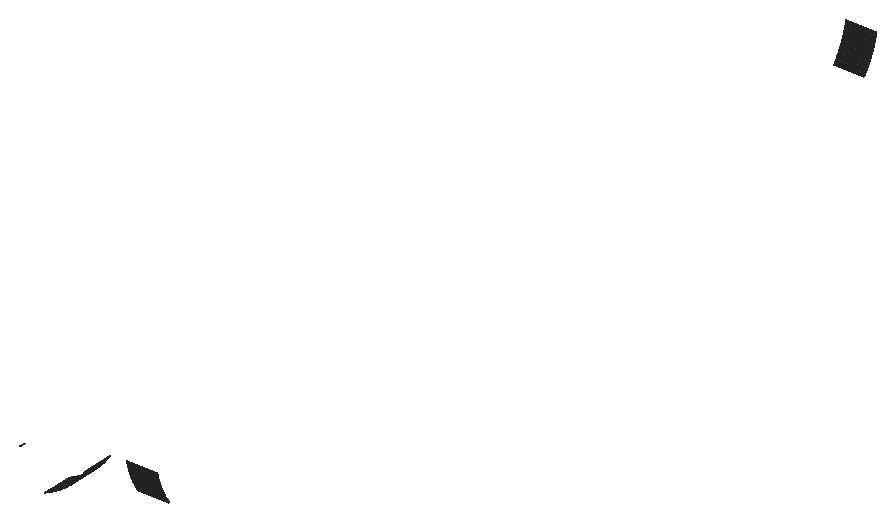
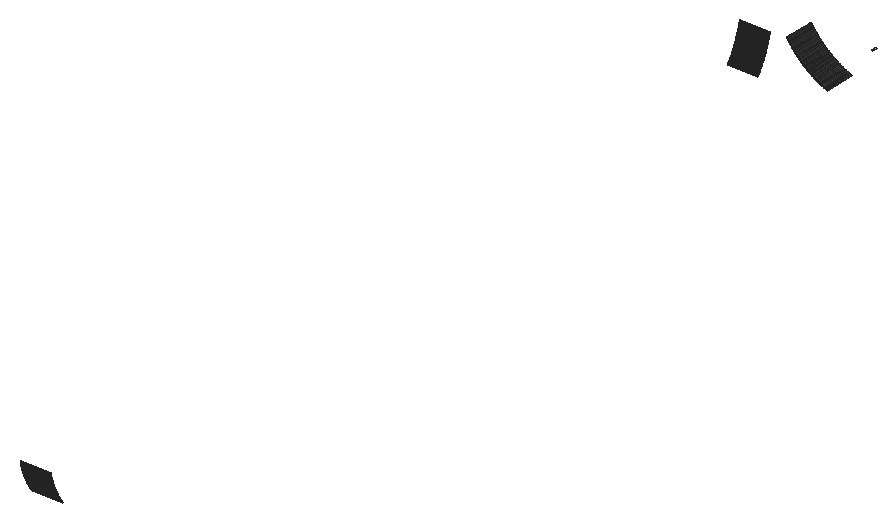
# SketchUp Ruby script. Lengths in inches.
U = 1.inch
M = Sketchup.active_model
def pt(a) = Geom::Point3d.new(a.map { |v| v * U })
def face(e, loops, mat)
  f = e.add_face(loops[0].map { |a| pt(a) })
  loops[1..].each { |l| e.add_face(l.map { |a| pt(a) }).erase! }
  f.material = f.back_material = mat if mat
  f
end
# faces: each face lists its corners as indices into pts; further lists are holes
def faces(e, pts, list, mat = nil) = list.each { |f| face(e, (f[0].is_a?(Array) ? f : [f]).map { |l| l.map { |i| pts[i] } }, mat) }
# xy, xz, yz: faces in a plane at the given z, y or x. An outline is a flat list of corners, or four numbers for a rectangle; further outlines are holes
def ring(l) = l.size == 4 ? [[l[0], l[1]], [l[2], l[1]], [l[2], l[3]], [l[0], l[3]]] : l.each_slice(2).to_a
def flat(e, list, mat, &to3) = list.each { |f| face(e, (f[0].is_a?(Array) ? f : [f]).map { |l| ring(l).map { |u, v| to3.(u, v) } }, mat) }
def xy(e, z, list, mat = nil) = flat(e, list, mat) { |x, y| [x, y, z] }
def xz(e, y, list, mat = nil) = flat(e, list, mat) { |x, z| [x, y, z] }
def yz(e, x, list, mat = nil) = flat(e, list, mat) { |y, z| [x, y, z] }
def lines(e, pts, list) = list.each { |a, b| e.add_line(pt(pts[a]), pt(pts[b])) }
# prism: a flat outline (further loops are holes) pulled along v
def prism(e, loops, v, mat = nil)
  f = face(e, loops, mat); d = Geom::Vector3d.new(v.map { |x| x * U })
  f.pushpull(f.normal.samedirection?(d) ? d.length : -d.length)
end
def box(e, o, s, mat = nil) = prism(e, [[o, [o[0] + s[0], o[1], o[2]], [o[0] + s[0], o[1] + s[1], o[2]], [o[0], o[1] + s[1], o[2]]]], [0, 0, s[2]], mat)
def at(x, y, z, deg = 0) = Geom::Transformation.translation(pt([x, y, z])) * Geom::Transformation.rotation(ORIGIN, Z_AXIS, deg.degrees)
def axes(o, x, y, z) = Geom::Transformation.new([*x, 0, *y, 0, *z, 0, *pt(o).to_a, 1])
def part(name) = M.definitions.add(name)
# library, detail: a bought-in or finely detailed component or shape, given as its bounding box
def library(name, o, s) = part(name).tap { |d| box(d.entities, o, s) }
def detail(e, o, s) = box(e.add_group.entities, o, s)
def put(e, d, t, mat = nil) = e.add_instance(d, t).tap { |i| i.material = mat if mat }
def group(e, t, mat = nil) = e.add_group.tap { |g| g.transformation = t; g.material = mat if mat }.entities
root = M.entities
M.materials.add("1432 AP 8245 TAR ROAD").color = [71, 72, 75]
M.materials.add("Outer Light").color = [251, 217, 152]
p = [[550.51,107.37,158.43],[550.78,107.37,158.53],[550.78,95.37,158.53],[550.51,95.37,158.43],[551.04,107.37,158.64],[551.04,95.37,158.64],
  [551.3,107.37,158.75],[551.3,95.37,158.75],[573,114.08,158.86],[573,114.25,158.63],[585,114.25,158.63],[585,114.08,158.86],
  [573,460.49,158.63],[573,460.66,158.86],[585,460.66,158.86],[585,460.49,158.63],[551.56,107.37,158.87],[551.56,95.37,158.87],
  [551.81,107.37,158.98],[551.81,95.37,158.98],[573,113.92,159.09],[585,113.92,159.09],[573,460.82,159.09],[585,460.82,159.09],
  [552.07,107.37,159.1],[552.07,95.37,159.1],[552.33,107.37,159.22],[552.33,95.37,159.22],[573,113.75,159.32],[585,113.75,159.32],
  [573,460.98,159.32],[585,460.98,159.32],[552.58,107.37,159.34],[552.58,95.37,159.34],[552.84,107.37,159.46],[552.84,95.37,159.46],
  [573,113.6,159.56],[585,113.6,159.56],[573,461.14,159.56],[585,461.14,159.56],[553.09,107.37,159.59],[553.09,95.37,159.59],
  [553.34,107.37,159.72],[553.34,95.37,159.72],[573,113.4375,159.79],[585,113.4375,159.79],[573,461.3,159.79],[585,461.3,159.79],
  [553.6,107.37,159.85],[553.6,95.37,159.85],[553.85,107.37,159.98],[553.85,95.37,159.98],[573,113.28,160.03],[585,113.28,160.03],
  [573,461.46,160.03],[585,461.46,160.03],[554.09,107.37,160.11],[554.09,95.37,160.11],[573,113.125,160.26],[585,113.125,160.26],
  [573,461.61,160.26],[585,461.61,160.26],[554.34,107.37,160.25],[554.34,95.37,160.25],[554.59,107.37,160.38],[554.59,95.37,160.38],
  [573,112.97,160.5],[585,112.97,160.5],[573,461.77,160.5],[585,461.77,160.5],[554.84,107.37,160.52],[554.84,95.37,160.52],
  [555.08,107.37,160.66],[555.08,95.37,160.66],[573,112.82,160.74],[585,112.82,160.74],[573,461.92,160.74],[585,461.92,160.74],
  [555.33,107.37,160.81],[555.33,95.37,160.81],[573,112.67,160.98],[585,112.67,160.98],[573,462.06,160.98],[585,462.06,160.98],
  [555.57,107.37,160.95],[555.57,95.37,160.95],[555.81,107.37,161.1],[555.81,95.37,161.1],[573,112.53,161.22],[585,112.53,161.22],
  [573,462.21,161.22],[585,462.21,161.22],[556.05,107.37,161.25],[556.05,95.37,161.25],[556.29,107.37,161.4],[556.29,95.37,161.4],
  [573,112.38,161.47],[585,112.38,161.47],[573,462.36,161.47],[585,462.36,161.47],[556.53,107.37,161.55],[556.53,95.37,161.55],
  [556.76,107.37,161.7],[556.76,95.37,161.7],[573,112.24,161.71],[585,112.24,161.71],[573,462.5,161.71],[585,462.5,161.71],
  [557,107.37,161.86],[557,95.37,161.86],[573,112.1,161.96],[585,112.1,161.96],[573,462.64,161.96],[585,462.64,161.96],
  [557.24,107.37,162.02],[557.24,95.37,162.02],[557.47,107.37,162.18],[557.47,95.37,162.18],[573,111.96,162.2],[585,111.96,162.2],
  [573,462.78,162.2],[585,462.78,162.2],[557.7,107.37,162.34],[557.7,95.37,162.34],[573,111.82,162.45],[585,111.82,162.45],
  [573,462.92,162.45],[585,462.92,162.45],[557.93,107.37,162.5],[557.93,95.37,162.5],[573,111.6875,162.7],[585,111.6875,162.7],
  [573,463.05,162.7],[585,463.05,162.7],[558.16,107.37,162.67],[558.16,95.37,162.67],[558.39,107.37,162.83],[558.39,95.37,162.83],
  [573,111.55,162.95],[585,111.55,162.95],[573,463.19,162.95],[585,463.19,162.95],[558.62,107.37,163],[558.62,95.37,163],
  [573,111.42,163.2],[585,111.42,163.2],[573,463.32,163.2],[585,463.32,163.2],[558.84,107.37,163.17],[558.84,95.37,163.17],
  [559.06,107.37,163.35],[559.06,95.37,163.35],[573,111.29,163.45],[585,111.29,163.45],[573,463.45,163.45],[585,463.45,163.45],
  [559.29,107.37,163.52],[559.29,95.37,163.52],[573,111.17,163.7],[585,111.17,163.7],[573,463.57,163.7],[585,463.57,163.7],
  [559.51,107.37,163.7],[559.51,95.37,163.7],[559.73,107.37,163.875],[559.73,95.37,163.875],[573,111.04,163.95],[585,111.04,163.95],
  [573,463.7,163.95],[585,463.7,163.95],[559.95,107.37,164.05],[559.95,95.37,164.05],[573,110.92,164.21],[585,110.92,164.21],
  [573,463.82,164.21],[585,463.82,164.21],[560.16,107.37,164.23],[560.16,95.37,164.23],[560.38,107.37,164.42],[560.38,95.37,164.42],
  [573,110.8,164.46],[585,110.8,164.46],[573,463.94,164.46],[585,463.94,164.46],[560.59,107.37,164.6],[560.59,95.37,164.6],
  [573,110.68,164.72],[585,110.68,164.72],[573,464.0625,164.72],[585,464.0625,164.72],[560.81,107.37,164.79],[560.81,95.37,164.79],
  [573,110.56,164.98],[585,110.56,164.98],[573,464.18,164.98],[585,464.18,164.98],[561.02,107.37,164.98],[561.02,95.37,164.98],
  [561.23,107.37,165.17],[561.23,95.37,165.17],[573,110.44,165.24],[585,110.44,165.24],[573,464.3,165.24],[585,464.3,165.24],
  [561.4375,107.37,165.36],[561.4375,95.37,165.36],[573,110.33,165.49],[585,110.33,165.49],[573,464.41,165.49],[585,464.41,165.49],
  [561.64,107.37,165.55],[561.64,95.37,165.55],[561.85,107.37,165.74],[561.85,95.37,165.74],[573,110.22,165.75],[585,110.22,165.75],
  [573,464.52,165.75],[585,464.52,165.75],[562.05,107.37,165.94],[562.05,95.37,165.94],[573,110.11,166.02],[585,110.11,166.02],
  [573,464.63,166.02],[585,464.63,166.02],[562.26,107.37,166.14],[562.26,95.37,166.14],[573,110,166.28],[585,110,166.28],
  [573,464.74,166.28],[585,464.74,166.28],[562.46,107.37,166.34],[562.46,95.37,166.34],[562.65,107.37,166.54],[562.65,95.37,166.54],
  [573,109.9,166.54],[585,109.9,166.54],[573,464.84,166.54],[585,464.84,166.54],[562.85,107.37,166.74],[562.85,95.37,166.74],
  [573,109.79,166.8],[585,109.79,166.8],[573,464.94,166.8],[585,464.94,166.8],[563.05,107.37,166.94],[563.05,95.37,166.94],
  [573,109.69,167.07],[585,109.69,167.07],[573,465.05,167.07],[585,465.05,167.07],[563.24,107.37,167.15],[563.24,95.37,167.15],
  [563.4375,107.37,167.36],[563.4375,95.37,167.36],[573,109.6,167.33],[585,109.6,167.33],[573,465.14,167.33],[585,465.14,167.33],
  [573,109.5,167.6],[585,109.5,167.6],[573,465.24,167.6],[585,465.24,167.6],[563.625,107.37,167.5625],[563.625,95.37,167.5625],
  [563.82,107.37,167.77],[563.82,95.37,167.77],[573,109.4,167.86],[585,109.4,167.86],[573,465.34,167.86],[585,465.34,167.86],
  [564,107.37,167.98],[564,95.37,167.98],[573,109.3125,168.13],[585,109.3125,168.13],[573,465.43,168.13],[585,465.43,168.13],
  [564.19,107.37,168.2],[564.19,95.37,168.2],[573,109.22,168.4],[585,109.22,168.4],[573,465.52,168.4],[585,465.52,168.4],
  [564.375,107.37,168.41],[564.375,95.37,168.41],[564.56,107.37,168.63],[564.56,95.37,168.63],[573,109.13,168.67],[585,109.13,168.67],
  [573,465.61,168.67],[585,465.61,168.67],[564.74,107.37,168.84],[564.74,95.37,168.84],[573,109.05,168.9375],[585,109.05,168.9375],
  [573,465.69,168.9375],[585,465.69,168.9375],[564.92,107.37,169.0625],[564.92,95.37,169.0625],[573,108.96,169.21],[585,108.96,169.21],
  [573,465.78,169.21],[585,465.78,169.21],[565.1,107.37,169.28],[565.1,95.37,169.28],[573,108.88,169.48],[585,108.88,169.48],
  [573,465.86,169.48],[585,465.86,169.48],[565.27,107.37,169.5],[565.27,95.37,169.5],[565.45,107.37,169.73],[565.45,95.37,169.73],
  [573,108.8,169.75],[585,108.8,169.75],[573,465.94,169.75],[585,465.94,169.75],[565.62,107.37,169.95],[565.62,95.37,169.95],
  [573,108.72,170.02],[585,108.72,170.02],[573,466.02,170.02],[585,466.02,170.02],[565.79,107.37,170.18],[565.79,95.37,170.18],
  [573,108.65,170.29],[585,108.65,170.29],[573,466.09,170.29],[585,466.09,170.29],[565.96,107.37,170.4],[565.96,95.37,170.4],
  [573,108.57,170.57],[585,108.57,170.57],[573,466.17,170.57],[585,466.17,170.57],[566.125,107.37,170.63],[566.125,95.37,170.63],
  [566.29,107.37,170.86],[566.29,95.37,170.86],[573,108.5,170.84],[585,108.5,170.84],[573,466.24,170.84],[585,466.24,170.84],
  [573,108.43,171.11],[585,108.43,171.11],[573,466.31,171.11],[585,466.31,171.11],[566.45,107.37,171.09],[566.45,95.37,171.09],
  [566.62,107.37,171.32],[566.62,95.37,171.32],[573,108.36,171.39],[585,108.36,171.39],[573,466.375,171.39],[585,466.375,171.39],
  [566.77,107.37,171.56],[566.77,95.37,171.56],[573,108.3,171.66],[585,108.3,171.66],[573,466.44,171.66],[585,466.44,171.66],
  [566.93,107.37,171.79],[566.93,95.37,171.79],[540.84,96.87,171.66],[541,96.87,171.6875],[541,95.37,171.6875],[540.84,95.37,171.66],
  [541.16,96.87,171.72],[541.16,95.37,171.72],[541,95.37,171.6875],[541.16,95.37,171.72],[541.16,96.87,171.72],[541,96.87,171.6875],
  [541.31,96.87,171.75],[541.31,95.37,171.75],[541.31,95.37,171.75],[541.31,96.87,171.75],[573,108.24,171.9375],[585,108.24,171.9375],
  [573,466.5,171.9375],[585,466.5,171.9375]]
faces(root,p,[[0,1,2,3],[1,4,5,2],[4,6,7,5],[8,9,10,11],[12,13,14,15],[6,16,17,7],[16,18,19,17],[20,8,11,21],
  [13,22,23,14],[18,24,25,19],[24,26,27,25],[28,20,21,29],[22,30,31,23],[26,32,33,27],[32,34,35,33],[36,28,29,37],
  [30,38,39,31],[34,40,41,35],[40,42,43,41],[44,36,37,45],[38,46,47,39],[42,48,49,43],[48,50,51,49],[52,44,45,53],
  [46,54,55,47],[50,56,57,51],[58,52,53,59],[54,60,61,55],[56,62,63,57],[62,64,65,63],[66,58,59,67],[60,68,69,61],
  [64,70,71,65],[70,72,73,71],[74,66,67,75],[68,76,77,69],[72,78,79,73],[80,74,75,81],[76,82,83,77],[78,84,85,79],
  [84,86,87,85],[88,80,81,89],[82,90,91,83],[86,92,93,87],[92,94,95,93],[96,88,89,97],[90,98,99,91],[94,100,101,95],
  [100,102,103,101],[104,96,97,105],[98,106,107,99],[102,108,109,103],[110,104,105,111],[106,112,113,107],[108,114,115,109],[114,116,117,115],
  [118,110,111,119],[112,120,121,113],[116,122,123,117],[124,118,119,125],[120,126,127,121],[122,128,129,123],[130,124,125,131],[126,132,133,127],
  [128,134,135,129],[134,136,137,135],[138,130,131,139],[132,140,141,133],[136,142,143,137],[144,138,139,145],[140,146,147,141],[142,148,149,143],
  [148,150,151,149],[152,144,145,153],[146,154,155,147],[150,156,157,151],[158,152,153,159],[154,160,161,155],[156,162,163,157],[162,164,165,163],
  [166,158,159,167],[160,168,169,161],[164,170,171,165],[172,166,167,173],[168,174,175,169],[170,176,177,171],[176,178,179,177],[180,172,173,181],
  [174,182,183,175],[178,184,185,179],[186,180,181,187],[182,188,189,183],[184,190,191,185],[192,186,187,193],[188,194,195,189],[190,196,197,191],
  [196,198,199,197],[200,192,193,201],[194,202,203,195],[198,204,205,199],[206,200,201,207],[202,208,209,203],[204,210,211,205],[210,212,213,211],
  [214,206,207,215],[208,216,217,209],[212,218,219,213],[220,214,215,221],[216,222,223,217],[218,224,225,219],[226,220,221,227],[222,228,229,223],
  [224,230,231,225],[230,232,233,231],[234,226,227,235],[228,236,237,229],[232,238,239,233],[240,234,235,241],[236,242,243,237],[238,244,245,239],
  [246,240,241,247],[242,248,249,243],[244,250,251,245],[250,252,253,251],[254,246,247,255],[248,256,257,249],[258,254,255,259],[256,260,261,257],
  [252,262,263,253],[262,264,265,263],[266,258,259,267],[260,268,269,261],[264,270,271,265],[272,266,267,273],[268,274,275,269],[270,276,277,271],
  [278,272,273,279],[274,280,281,275],[276,282,283,277],[282,284,285,283],[286,278,279,287],[280,288,289,281],[284,290,291,285],[292,286,287,293],
  [288,294,295,289],[290,296,297,291],[298,292,293,299],[294,300,301,295],[296,302,303,297],[304,298,299,305],[300,306,307,301],[302,308,309,303],
  [308,310,311,309],[312,304,305,313],[306,314,315,307],[310,316,317,311],[318,312,313,319],[314,320,321,315],[316,322,323,317],[324,318,319,325],
  [320,326,327,321],[322,328,329,323],[330,324,325,331],[326,332,333,327],[328,334,335,329],[334,336,337,335],[338,330,331,339],[332,340,341,333],
  [342,338,339,343],[340,344,345,341],[336,346,347,337],[346,348,349,347],[350,342,343,351],[344,352,353,345],[348,354,355,349],[356,350,351,357],
  [352,358,359,353],[354,360,361,355],[368,369,370,371],[369,374,375,370],[376,356,357,377],[358,378,379,359]],"1432 AP 8245 TAR ROAD")
faces(root,p,[[362,363,364,365],[363,366,367,364],[366,372,373,367]],"Outer Light")
